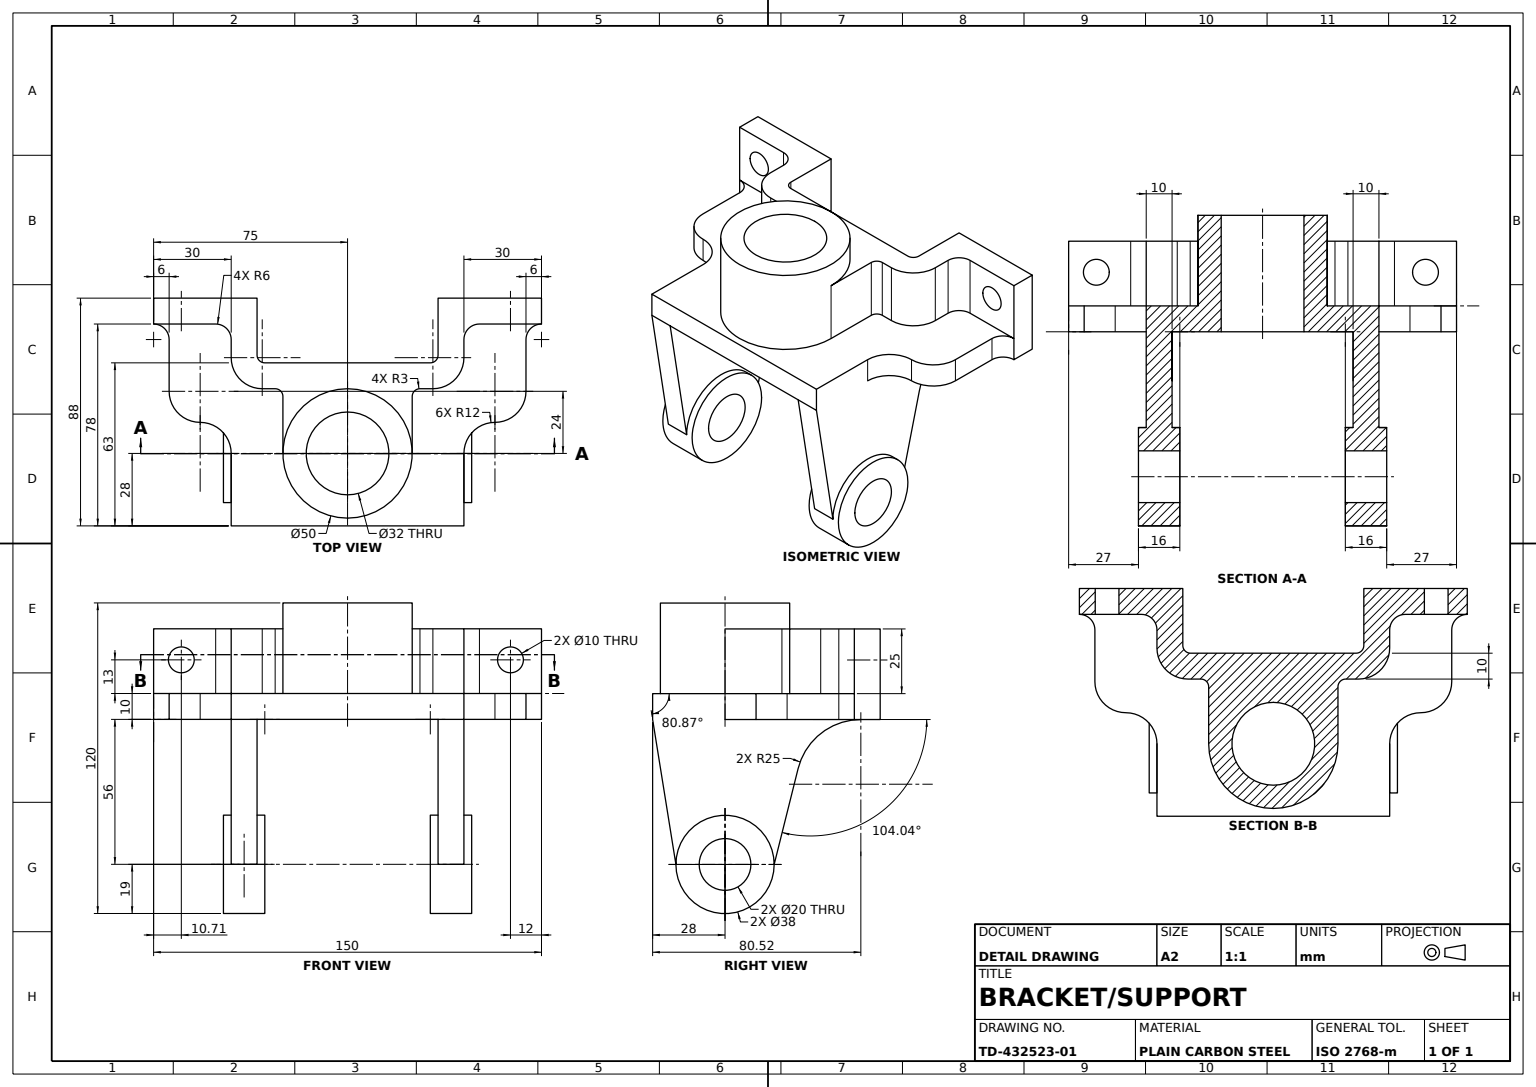
solid
v1 (69,10,-72)
v2 (75,10,-78)
e1 v1 v2 CIRCLE(AX(P(75,10,-72),D(0,-1,0),D(0,0,-1)),6)
v3 (69,0,-72)
e2 v3 v1 LINE
v4 (75,0,-78)
e3 v4 v3 CIRCLE(AX(P(75,0,-72),D(0,1,0),D(0,0,-1)),6)
e4 v2 v4 LINE
face CYL(AX(P(75,10,-72),D(0,1,0),D(0,0,1)),6) rev [-e1 -e2 -e3 -e4]
v5 (35,0,0)
v6 (45,0,0)
e5 v5 v6 LINE
v7 (45,10,0)
e6 v7 v6 LINE
v8 (-45,10,0)
e7 v8 v7 LINE
v9 (-45,0,0)
e8 v8 v9 LINE
v10 (-35,0,0)
e9 v9 v10 LINE
e10 v10 v5 LINE
face PLANE(AX(P(0,10,0),D(0,0,-1),D(-1,0,0))) rev [e5 -e6 -e7 e8 e9 e10]
v11 (-32,-56,-47)
v12 (-35,-56,-47)
e11 v11 v12 LINE
v13 (-32,-56,-9)
e12 v13 v11 CIRCLE(AX(P(-32,-56,-28),D(1,0,0),D(0,0,-1)),19)
v14 (-35,-56,-9)
e13 v13 v14 LINE
v15 (-45,-56,-9)
e14 v14 v15 LINE
v16 (-48,-56,-9)
e15 v15 v16 LINE
v17 (-48,-56,-47)
e16 v17 v16 CIRCLE(AX(P(-48,-56,-28),D(-1,0,0),D(0,0,1)),19)
v18 (-45,-56,-47)
e17 v18 v17 LINE
e18 v12 v18 LINE
face CYL(AX(P(-35,-56,-28),D(-1,0,0),D(0,0,1)),19) [-e11 -e12 e13 e14 e15 -e16 -e17 -e18]
v19 (75,0,-88)
v20 (35,0,-88)
e19 v19 v20 LINE
e20 v4 v19 LINE
v21 (69,0,-52)
e21 v21 v3 LINE
v22 (57,0,-40)
e22 v21 v22 CIRCLE(AX(P(57,0,-52),D(0,-1,0),D(0,0,-1)),12)
v23 (45,0,-28)
e23 v23 v22 CIRCLE(AX(P(57,0,-28),D(0,-1,0),D(0,0,-1)),12)
v24 (45,0,-80.51941)
e24 v24 v23 LINE
v25 (35,0,-80.51941)
e25 v25 v24 LINE
e26 v20 v25 LINE
face PLANE(AX(P(57,0,-28),D(0,-1,0),D(0,0,-1))) [-e19 -e20 e3 -e21 e22 -e23 -e24 -e25 -e26]
v26 (45,35,-65)
v27 (45,35,-72)
e27 v26 v27 LINE
v28 (45,10,-65)
e28 v26 v28 LINE
v29 (45,10,-72)
e29 v28 v29 LINE
e30 v27 v29 LINE
face PLANE(AX(P(45,35,0),D(-1,0,0),D(0,0,1))) rev [-e27 e28 e29 -e30]
v30 (-25,10,-28)
v31 (0,10,-3)
e31 v30 v31 CIRCLE(AX(P(0,10,-28),D(0,1,0),D(0,0,1)),25)
v32 (0,45,-3)
e32 v32 v31 LINE
v33 (0,45,-53)
e33 v33 v32 CIRCLE(AX(P(0,45,-28),D(0,1,0),D(0,0,1)),25)
v34 (0,35,-53)
e34 v33 v34 LINE
v35 (-25,35,-28)
e35 v34 v35 CIRCLE(AX(P(0,35,-28),D(0,1,0),D(0,0,1)),25)
e36 v35 v30 LINE
face CYL(AX(P(0,35,-28),D(0,-1,0),D(0,0,-1)),25) [e31 -e32 -e33 e34 e35 e36]
v36 (45,10,-28)
e37 v7 v36 LINE
v37 (45,-56,-9)
e38 v37 v6 LINE
v38 (45,-56,-47)
e39 v38 v37 CIRCLE(AX(P(45,-56,-28),D(1,0,0),D(0,0,-1)),19)
v39 (45,-18.936609,-56.265848)
e40 v39 v38 LINE
e41 v24 v39 CIRCLE(AX(P(45,-25,-80.51941),D(1,0,0),D(0,0,-1)),25)
e42 v36 v23 LINE
face PLANE(AX(P(45,10,0),D(-1,0,0),D(0,0,1))) rev [-e37 e6 -e38 -e39 -e40 -e41 e24 -e42]
v40 (-75,0,-88)
v41 (-75,0,-78)
e43 v40 v41 LINE
v42 (-75,10,-78)
e44 v42 v41 LINE
v43 (-75,35,-78)
e45 v43 v42 LINE
v44 (-75,35,-88)
e46 v44 v43 LINE
e47 v44 v40 LINE
face PLANE(AX(P(-75,10,-88),D(1,0,0),D(0,0,-1))) rev [e43 -e44 -e45 -e46 e47]
v45 (-57,0,-40)
v46 (-69,0,-52)
e48 v45 v46 CIRCLE(AX(P(-57,0,-52),D(0,-1,0),D(0,0,-1)),12)
v47 (-69,0,-72)
e49 v47 v46 LINE
e50 v47 v41 CIRCLE(AX(P(-75,0,-72),D(0,1,0),D(0,0,-1)),6)
v48 (-35,0,-88)
e51 v48 v40 LINE
v49 (-35,0,-80.51941)
e52 v49 v48 LINE
v50 (-45,0,-80.51941)
e53 v49 v50 LINE
v51 (-45,0,-28)
e54 v50 v51 LINE
e55 v45 v51 CIRCLE(AX(P(-57,0,-28),D(0,-1,0),D(0,0,-1)),12)
face PLANE(AX(P(57,0,-28),D(0,-1,0),D(0,0,-1))) [e48 -e49 e50 -e43 -e51 -e52 e53 e54 -e55]
v52 (-32,-56,-18)
v53 (-32,-56,-38)
e56 v52 v53 CIRCLE(AX(P(-32,-56,-28),D(1,0,0),D(0,0,-1)),10)
v54 (-48,-56,-38)
e57 v53 v54 LINE
v55 (-48,-56,-18)
e58 v54 v55 CIRCLE(AX(P(-48,-56,-28),D(-1,0,0),D(0,0,1)),10)
e59 v52 v55 LINE
face CYL(AX(P(67,-56,-28),D(-1,0,0),D(0,0,1)),10) rev [e56 e57 e58 -e59]
e60 v11 v13 CIRCLE(AX(P(-32,-56,-28),D(1,0,0),D(0,0,-1)),19)
e61 v53 v52 CIRCLE(AX(P(-32,-56,-28),D(1,0,0),D(0,0,-1)),10)
face PLANE(AX(P(-32,-56,-28),D(1,0,0),D(0,0,-1))) [e12 e60] [-e61 -e56]
v56 (-51,10,-78)
e62 v56 v42 LINE
v57 (-51,35,-78)
e63 v57 v56 LINE
e64 v57 v43 LINE
v58 (-59.287205,23,-78)
v59 (-69.287205,23,-78)
e65 v58 v59 CIRCLE(AX(P(-64.287205,23,-78),D(0,0,1),D(1,0,0)),5)
e66 v59 v58 CIRCLE(AX(P(-64.287205,23,-78),D(0,0,1),D(1,0,0)),5)
face PLANE(AX(P(0,35,-78),D(0,0,1),D(1,0,0))) [-e62 -e63 e64 e45] [-e65 -e66]
v60 (-28,35,-53)
v61 (-28,10,-53)
e67 v60 v61 LINE
v62 (-33,35,-53)
e68 v60 v62 LINE
v63 (-33,10,-53)
e69 v62 v63 LINE
e70 v61 v63 LINE
face PLANE(AX(P(0,35,-53),D(0,0,1),D(1,0,0))) [-e67 e68 e69 -e70]
v64 (-45,-18.936609,-56.265848)
e71 v50 v64 CIRCLE(AX(P(-45,-25,-80.51941),D(1,0,0),D(0,0,1)),25)
e72 v64 v18 LINE
e73 v15 v18 CIRCLE(AX(P(-45,-56,-28),D(-1,0,0),D(0,0,1)),19)
e74 v15 v9 LINE
v65 (-45,10,-28)
e75 v65 v8 LINE
e76 v65 v51 LINE
face PLANE(AX(P(-45,10,-28),D(1,0,0),D(0,0,-1))) rev [e71 e72 -e73 e74 -e8 -e75 e76 -e54]
v66 (33,35,-53)
e77 v66 v26 CIRCLE(AX(P(33,35,-65),D(0,1,0),D(0,0,1)),12)
v67 (33,10,-53)
e78 v66 v67 LINE
e79 v67 v28 CIRCLE(AX(P(33,10,-65),D(0,1,0),D(0,0,1)),12)
face CYL(AX(P(33,35,-65),D(0,-1,0),D(0,0,-1)),12) [-e77 e78 e79 -e28]
v68 (35,35,-66)
v69 (32,35,-63)
e80 v68 v69 CIRCLE(AX(P(32,35,-66),D(0,-1,0),D(0,0,1)),3)
v70 (35,0,-66)
e81 v68 v70 LINE
v71 (32,0,-63)
e82 v70 v71 CIRCLE(AX(P(32,0,-66),D(0,-1,0),D(0,0,-1)),3)
e83 v69 v71 LINE
face CYL(AX(P(32,10,-66),D(0,-1,0),D(0,0,-1)),3) rev [-e80 e81 e82 -e83]
v72 (57,10,-40)
e84 v72 v22 LINE
e85 v36 v72 CIRCLE(AX(P(57,10,-28),D(0,-1,0),D(0,0,-1)),12)
face CYL(AX(P(57,10,-28),D(0,-1,0),D(0,0,-1)),12) rev [e23 -e84 -e85 e42]
v73 (28,35,-53)
e86 v73 v66 LINE
v74 (28,10,-53)
e87 v73 v74 LINE
e88 v74 v67 LINE
face PLANE(AX(P(0,35,-53),D(0,0,-1),D(-1,0,0))) rev [-e86 e87 e88 -e78]
v75 (69,10,-52)
e89 v72 v75 CIRCLE(AX(P(57,10,-52),D(0,1,0),D(0,0,-1)),12)
e90 v75 v21 LINE
face CYL(AX(P(57,10,-52),D(0,-1,0),D(0,0,-1)),12) [-e89 e84 -e22 -e90]
v76 (51,35,-78)
v77 (75,35,-78)
e91 v76 v77 LINE
v78 (75,35,-88)
e92 v77 v78 LINE
v79 (35,35,-88)
e93 v78 v79 LINE
e94 v79 v68 LINE
v80 (-32,35,-63)
e95 v69 v80 LINE
v81 (-35,35,-66)
e96 v80 v81 CIRCLE(AX(P(-32,35,-66),D(0,-1,0),D(0,0,1)),3)
v82 (-35,35,-88)
e97 v81 v82 LINE
e98 v82 v44 LINE
v83 (-45,35,-72)
e99 v83 v57 CIRCLE(AX(P(-51,35,-72),D(0,1,0),D(0,0,1)),6)
v84 (-45,35,-65)
e100 v84 v83 LINE
e101 v62 v84 CIRCLE(AX(P(-33,35,-65),D(0,-1,0),D(0,0,1)),12)
v85 (-25,35,-50)
e102 v85 v60 CIRCLE(AX(P(-28,35,-50),D(0,1,0),D(0,0,1)),3)
e103 v35 v85 LINE
v86 (25,35,-28)
e104 v86 v34 CIRCLE(AX(P(0,35,-28),D(0,1,0),D(0,0,1)),25)
v87 (25,35,-50)
e105 v86 v87 LINE
e106 v87 v73 CIRCLE(AX(P(28,35,-50),D(0,-1,0),D(0,0,1)),3)
e107 v27 v76 CIRCLE(AX(P(51,35,-72),D(0,-1,0),D(0,0,1)),6)
face PLANE(AX(P(0,35,0),D(0,1,0),D(0,0,1))) [e91 e92 e93 e94 e80 e95 e96 e97 e98 e46 -e64 -e99 -e100 -e101 -e68 -e102 -e103 -e35 -e104 e105 e106 e86 e77 e27 e107]
v88 (0,0,-12)
v89 (0,45,-12)
e108 v88 v89 LINE
v90 (0,0,-44)
e109 v88 v90 CIRCLE(AX(P(0,0,-28),D(0,-1,0),D(0,0,-1)),16)
v91 (0,45,-44)
e110 v90 v91 LINE
e111 v91 v89 CIRCLE(AX(P(0,45,-28),D(0,1,0),D(0,0,1)),16)
face CYL(AX(P(0,-217,-28),D(0,1,0),D(0,0,1)),16) rev [-e108 e109 e110 e111]
v92 (35,-56,-9)
v93 (35,-56,-47)
e112 v92 v93 CIRCLE(AX(P(35,-56,-28),D(-1,0,0),D(0,0,1)),19)
e113 v92 v5 LINE
e114 v5 v70 LINE
e115 v79 v20 LINE
v94 (35,-18.936609,-56.265848)
e116 v25 v94 CIRCLE(AX(P(35,-25,-80.51941),D(1,0,0),D(0,0,-1)),25)
e117 v94 v93 LINE
face PLANE(AX(P(35,10,-88),D(1,0,0),D(0,0,-1))) rev [-e112 e113 e114 -e81 -e94 e115 e26 e116 e117]
e118 v16 v17 CIRCLE(AX(P(-48,-56,-28),D(-1,0,0),D(0,0,1)),19)
face CYL(AX(P(-35,-56,-28),D(-1,0,0),D(0,0,1)),19) [-e118 -e15 e73 e17]
v95 (51,10,-78)
e119 v95 v2 LINE
e120 v29 v95 CIRCLE(AX(P(51,10,-72),D(0,-1,0),D(0,0,1)),6)
v96 (25,10,-50)
e121 v96 v74 CIRCLE(AX(P(28,10,-50),D(0,-1,0),D(0,0,1)),3)
v97 (25,10,-28)
e122 v97 v96 LINE
e123 v31 v97 CIRCLE(AX(P(0,10,-28),D(0,1,0),D(0,0,1)),25)
v98 (-25,10,-50)
e124 v30 v98 LINE
e125 v98 v61 CIRCLE(AX(P(-28,10,-50),D(0,1,0),D(0,0,1)),3)
v99 (-45,10,-65)
e126 v63 v99 CIRCLE(AX(P(-33,10,-65),D(0,-1,0),D(0,0,1)),12)
v100 (-45,10,-72)
e127 v99 v100 LINE
e128 v100 v56 CIRCLE(AX(P(-51,10,-72),D(0,1,0),D(0,0,1)),6)
v101 (-69,10,-72)
e129 v42 v101 CIRCLE(AX(P(-75,10,-72),D(0,-1,0),D(0,0,-1)),6)
v102 (-69,10,-52)
e130 v101 v102 LINE
v103 (-57,10,-40)
e131 v102 v103 CIRCLE(AX(P(-57,10,-52),D(0,1,0),D(0,0,-1)),12)
e132 v103 v65 CIRCLE(AX(P(-57,10,-28),D(0,-1,0),D(0,0,-1)),12)
e133 v75 v1 LINE
face PLANE(AX(P(57,10,-28),D(0,-1,0),D(0,0,-1))) rev [-e119 -e120 -e29 -e79 -e88 -e121 -e122 -e123 -e31 e124 e125 e70 e126 e127 e128 e62 e129 e130 e131 e132 e75 e7 e37 e85 e89 e133 e1]
e134 v14 v10 LINE
face PLANE(AX(P(-35,0,0),D(0,-0.158678095,0.987330371),D(0,-0.987330371,-0.158678095))) [-e14 e134 -e9 -e74]
e135 v92 v37 LINE
face PLANE(AX(P(35,0,0),D(0,0.158678095,-0.987330371),D(0,0.987330371,0.158678095))) rev [e38 -e5 -e113 e135]
e136 v76 v95 LINE
face CYL(AX(P(51,35,-72),D(0,-1,0),D(0,0,-1)),6) rev [e120 -e136 -e107 e30]
e137 v77 v2 LINE
e138 v78 v19 LINE
face PLANE(AX(P(75,10,-78),D(-1,0,0),D(0,0,1))) rev [e137 e4 e20 -e138 -e92]
v104 (-32,0,-63)
e139 v71 v104 LINE
e140 v80 v104 LINE
face PLANE(AX(P(32,10,-63),D(0,0,1),D(1,0,0))) rev [e83 e139 -e140 -e95]
e141 v55 v54 CIRCLE(AX(P(-48,-56,-28),D(-1,0,0),D(0,0,1)),10)
face CYL(AX(P(67,-56,-28),D(-1,0,0),D(0,0,1)),10) rev [e59 e141 -e57 e61]
e142 v89 v91 CIRCLE(AX(P(0,45,-28),D(0,1,0),D(0,0,1)),16)
e143 v90 v88 CIRCLE(AX(P(0,0,-28),D(0,-1,0),D(0,0,-1)),16)
face CYL(AX(P(0,-217,-28),D(0,1,0),D(0,0,1)),16) rev [e142 -e110 e143 e108]
v105 (48,-56,-9)
v106 (48,-56,-47)
e144 v105 v106 CIRCLE(AX(P(48,-56,-28),D(1,0,0),D(0,0,-1)),19)
e145 v106 v105 CIRCLE(AX(P(48,-56,-28),D(1,0,0),D(0,0,-1)),19)
v107 (48,-56,-38)
v108 (48,-56,-18)
e146 v107 v108 CIRCLE(AX(P(48,-56,-28),D(1,0,0),D(0,0,-1)),10)
e147 v108 v107 CIRCLE(AX(P(48,-56,-28),D(1,0,0),D(0,0,-1)),10)
face PLANE(AX(P(48,-56,-28),D(1,0,0),D(0,0,-1))) [e144 e145] [-e146 -e147]
e148 v84 v99 LINE
face CYL(AX(P(-33,35,-65),D(0,-1,0),D(0,0,-1)),12) [e148 -e126 -e69 e101]
e149 v46 v102 LINE
e150 v103 v45 LINE
face CYL(AX(P(-57,10,-52),D(0,-1,0),D(0,0,-1)),12) [-e131 -e149 -e48 -e150]
e151 v86 v97 LINE
e152 v32 v33 CIRCLE(AX(P(0,45,-28),D(0,1,0),D(0,0,1)),25)
face CYL(AX(P(0,35,-28),D(0,-1,0),D(0,0,-1)),25) [e32 e123 -e151 e104 -e34 -e152]
e153 v101 v47 LINE
face PLANE(AX(P(-69,10,-78),D(1,0,0),D(0,0,-1))) rev [e149 -e130 e153 e49]
v109 (58,23,-88)
v110 (68,23,-88)
e154 v109 v110 CIRCLE(AX(P(63,23,-88),D(0,0,1),D(1,0,0)),5)
v111 (58,23,-78)
e155 v109 v111 LINE
v112 (68,23,-78)
e156 v111 v112 CIRCLE(AX(P(63,23,-78),D(0,0,1),D(1,0,0)),5)
e157 v110 v112 LINE
face CYL(AX(P(63,23,-193),D(0,0,1),D(1,0,0)),5) rev [-e154 e155 e156 -e157]
e158 v87 v96 LINE
face PLANE(AX(P(25,35,0),D(-1,0,0),D(0,0,1))) rev [-e158 -e105 e151 e122]
face CYL(AX(P(28,35,-50),D(0,-1,0),D(0,0,-1)),3) rev [e158 e121 -e87 -e106]
e159 v83 v100 LINE
face CYL(AX(P(-51,35,-72),D(0,-1,0),D(0,0,-1)),6) rev [-e128 -e159 e99 e63]
v113 (32,-56,-18)
e160 v113 v108 LINE
v114 (32,-56,-38)
e161 v114 v107 LINE
e162 v114 v113 CIRCLE(AX(P(32,-56,-28),D(-1,0,0),D(0,0,1)),10)
face CYL(AX(P(-54,-56,-28),D(1,0,0),D(0,0,-1)),10) rev [e160 e147 -e161 e162]
v115 (-35,-18.936609,-56.265848)
e163 v115 v64 LINE
e164 v49 v115 CIRCLE(AX(P(-35,-25,-80.51941),D(1,0,0),D(0,0,1)),25)
face CYL(AX(P(-35,-25,-80.51941),D(-1,0,0),D(0,0,1)),25) rev [e163 -e71 -e53 e164]
e165 v93 v38 LINE
e166 v94 v39 LINE
face PLANE(AX(P(35,-14.352941,-57.411765),D(0,0.242535625,0.9701425),D(0,-0.9701425,0.242535625))) rev [e40 -e165 -e117 e166]
e167 v112 v111 CIRCLE(AX(P(63,23,-78),D(0,0,1),D(1,0,0)),5)
face PLANE(AX(P(0,35,-78),D(0,0,-1),D(-1,0,0))) rev [-e167 -e156] [-e91 e136 e119 -e137]
e168 v85 v98 LINE
face PLANE(AX(P(-25,35,0),D(-1,0,0),D(0,0,1))) [e168 -e124 -e36 e103]
v116 (-69.287205,23,-88)
e169 v116 v59 LINE
v117 (-59.287205,23,-88)
e170 v117 v116 CIRCLE(AX(P(-64.287205,23,-88),D(0,0,1),D(1,0,0)),5)
e171 v117 v58 LINE
face CYL(AX(P(-64.287205,23,-193),D(0,0,1),D(1,0,0)),5) rev [-e169 -e170 e171 e65]
face PLANE(AX(P(-45,35,0),D(-1,0,0),D(0,0,1))) [-e127 -e148 e100 e159]
face CYL(AX(P(-57,10,-28),D(0,-1,0),D(0,0,-1)),12) rev [-e132 e150 e55 -e76]
e172 v82 v48 LINE
e173 v116 v117 CIRCLE(AX(P(-64.287205,23,-88),D(0,0,1),D(1,0,0)),5)
face PLANE(AX(P(-35,10,-88),D(0,0,1),D(1,0,0))) rev [-e98 e172 e51 -e47] [e170 e173]
v118 (32,-56,-47)
e174 v118 v93 LINE
v119 (32,-56,-9)
e175 v119 v118 CIRCLE(AX(P(32,-56,-28),D(-1,0,0),D(0,0,1)),19)
e176 v119 v92 LINE
face CYL(AX(P(35,-56,-28),D(1,0,0),D(0,0,-1)),19) [e112 -e174 -e175 e176]
e177 v37 v105 LINE
e178 v38 v106 LINE
face CYL(AX(P(35,-56,-28),D(1,0,0),D(0,0,-1)),19) [e39 e177 -e145 -e178]
face CYL(AX(P(-28,35,-50),D(0,-1,0),D(0,0,-1)),3) rev [-e168 e102 e67 -e125]
face CYL(AX(P(35,-25,-80.51941),D(1,0,0),D(0,0,-1)),25) rev [e41 -e166 -e116 e25]
face CYL(AX(P(-64.287205,23,-193),D(0,0,1),D(1,0,0)),5) rev [e169 e66 -e171 -e173]
e179 v110 v109 CIRCLE(AX(P(63,23,-88),D(0,0,1),D(1,0,0)),5)
face CYL(AX(P(63,23,-193),D(0,0,1),D(1,0,0)),5) rev [-e179 e157 e167 -e155]
e180 v12 v14 CIRCLE(AX(P(-35,-56,-28),D(1,0,0),D(0,0,-1)),19)
face CYL(AX(P(-35,-56,-28),D(-1,0,0),D(0,0,1)),19) [e180 -e13 -e60 e11]
v120 (-35,0,-66)
e181 v104 v120 CIRCLE(AX(P(-32,0,-66),D(0,-1,0),D(0,0,-1)),3)
e182 v81 v120 LINE
face CYL(AX(P(-32,10,-66),D(0,-1,0),D(0,0,-1)),3) rev [-e96 e140 e181 -e182]
e183 v118 v119 CIRCLE(AX(P(32,-56,-28),D(-1,0,0),D(0,0,1)),19)
e184 v113 v114 CIRCLE(AX(P(32,-56,-28),D(-1,0,0),D(0,0,1)),10)
face PLANE(AX(P(32,-56,-28),D(-1,0,0),D(0,0,1))) [e175 e183] [-e184 -e162]
face PLANE(AX(P(-48,-56,-28),D(-1,0,0),D(0,0,1))) [-e141 -e58] [e16 e118]
face CYL(AX(P(35,-56,-28),D(1,0,0),D(0,0,-1)),19) [e174 e165 e178 -e144 -e177 -e135 -e176 -e183]
face CYL(AX(P(-75,10,-72),D(0,1,0),D(0,0,1)),6) rev [-e50 -e153 -e129 e44]
face PLANE(AX(P(0,45,-28),D(0,1,0),D(0,0,1))) [e152 e33] [-e111 -e142]
e185 v115 v12 LINE
e186 v120 v10 LINE
face PLANE(AX(P(-35,10,-66),D(-1,0,0),D(0,0,1))) rev [-e134 -e180 -e185 -e164 e52 -e172 -e97 e182 e186]
face CYL(AX(P(-54,-56,-28),D(1,0,0),D(0,0,-1)),10) rev [e161 e146 -e160 e184]
face PLANE(AX(P(57,0,-28),D(0,-1,0),D(0,0,-1))) [-e143 -e109] [-e10 -e186 -e181 -e139 -e82 -e114]
face PLANE(AX(P(-35,-14.352941,-57.411765),D(0,-0.242535625,-0.9701425),D(0,0.9701425,-0.242535625))) [-e72 -e163 e185 e18]
face PLANE(AX(P(69,10,-40),D(-1,0,0),D(0,0,1))) rev [e2 -e133 e90 e21]
face PLANE(AX(P(35,10,-88),D(0,0,1),D(1,0,0))) rev [e138 e19 -e115 -e93] [e154 e179]
